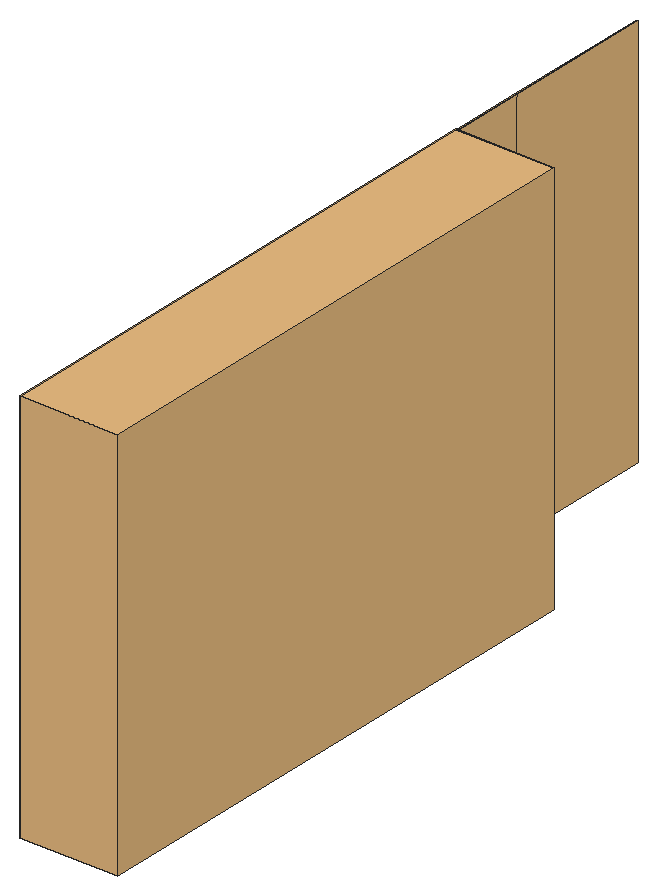
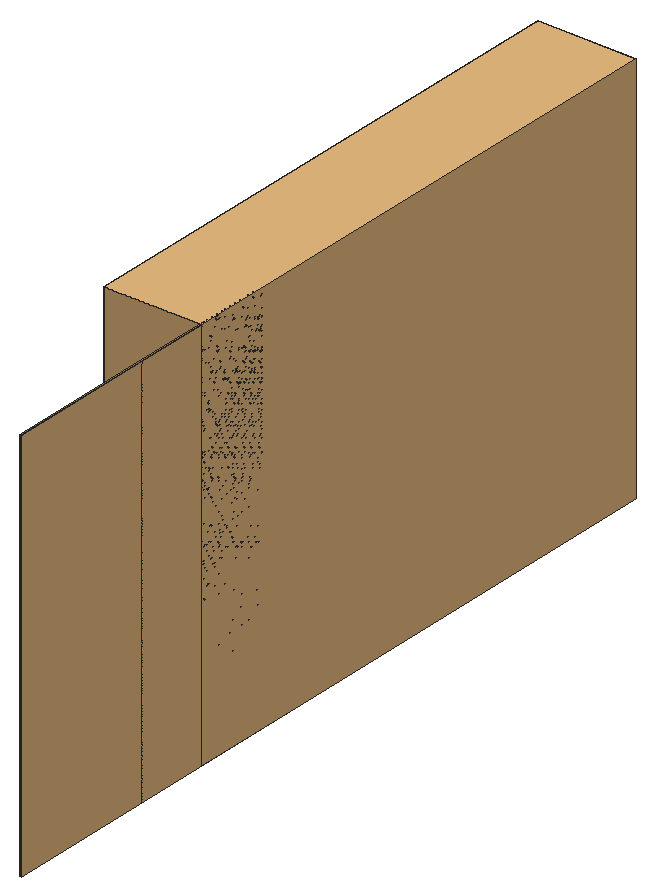
# SketchUp Ruby script. Lengths in inches.
U = 1.inch
M = Sketchup.active_model
def pt(a) = Geom::Point3d.new(a.map { |v| v * U })
def face(e, loops, mat)
  f = e.add_face(loops[0].map { |a| pt(a) })
  loops[1..].each { |l| e.add_face(l.map { |a| pt(a) }).erase! }
  f.material = f.back_material = mat if mat
  f
end
# faces: each face lists its corners as indices into pts; further lists are holes
def faces(e, pts, list, mat = nil) = list.each { |f| face(e, (f[0].is_a?(Array) ? f : [f]).map { |l| l.map { |i| pts[i] } }, mat) }
# xy, xz, yz: faces in a plane at the given z, y or x. An outline is a flat list of corners, or four numbers for a rectangle; further outlines are holes
def ring(l) = l.size == 4 ? [[l[0], l[1]], [l[2], l[1]], [l[2], l[3]], [l[0], l[3]]] : l.each_slice(2).to_a
def flat(e, list, mat, &to3) = list.each { |f| face(e, (f[0].is_a?(Array) ? f : [f]).map { |l| ring(l).map { |u, v| to3.(u, v) } }, mat) }
def xy(e, z, list, mat = nil) = flat(e, list, mat) { |x, y| [x, y, z] }
def xz(e, y, list, mat = nil) = flat(e, list, mat) { |x, z| [x, y, z] }
def yz(e, x, list, mat = nil) = flat(e, list, mat) { |y, z| [x, y, z] }
def lines(e, pts, list) = list.each { |a, b| e.add_line(pt(pts[a]), pt(pts[b])) }
# prism: a flat outline (further loops are holes) pulled along v
def prism(e, loops, v, mat = nil)
  f = face(e, loops, mat); d = Geom::Vector3d.new(v.map { |x| x * U })
  f.pushpull(f.normal.samedirection?(d) ? d.length : -d.length)
end
def box(e, o, s, mat = nil) = prism(e, [[o, [o[0] + s[0], o[1], o[2]], [o[0] + s[0], o[1] + s[1], o[2]], [o[0], o[1] + s[1], o[2]]]], [0, 0, s[2]], mat)
def at(x, y, z, deg = 0) = Geom::Transformation.translation(pt([x, y, z])) * Geom::Transformation.rotation(ORIGIN, Z_AXIS, deg.degrees)
def axes(o, x, y, z) = Geom::Transformation.new([*x, 0, *y, 0, *z, 0, *pt(o).to_a, 1])
def part(name) = M.definitions.add(name)
# library, detail: a bought-in or finely detailed component or shape, given as its bounding box
def library(name, o, s) = part(name).tap { |d| box(d.entities, o, s) }
def detail(e, o, s) = box(e.add_group.entities, o, s)
def put(e, d, t, mat = nil) = e.add_instance(d, t).tap { |i| i.material = mat if mat }
def group(e, t, mat = nil) = e.add_group.tap { |g| g.transformation = t; g.material = mat if mat }.entities
root = M.entities
M.materials.add("[Wood Veneer 01]").color = [120, 70, 37]
M.materials.add("green").color = [174, 139, 102]
M.materials.add("vio").color = [206, 114, 100]
c1 = library("3DGeom~53_Defintion",[-197.77,-500,-314.82],[395.54,1000,629.64])
c2 = part("3DGeom~54_Defintion")
p = [[-142.75,-484.5,-308.47],[-174.69,-472.9,-312.45],[-157.62,-477.6,-314.82],[-174.69,-472.9,-312.45],[-142.75,-484.5,-308.47],[-197.77,-474.24,-286.23],
  [-174.69,-472.9,-312.45],[-197.77,-474.24,-286.23],[-189.38,-471.68,-301.98],[-188.9,-487.18,-256.03],[-142.75,-484.5,-308.47],[-156.97,-498.77,-252.06],
  [-156.97,-498.77,-252.06],[-142.75,-484.5,-308.47],[-133.89,-497.43,-278.27],[-142.75,-484.5,-308.47],[-134.07,-491.76,-295.09],[-133.89,-497.43,-278.27],
  [-197.77,-474.24,-286.23],[-142.75,-484.5,-308.47],[-188.9,-487.18,-256.03],[-197.77,-474.24,-286.23],[-188.9,-487.18,-256.03],[-197.59,-479.92,-269.41],
  [-156.97,-498.77,-252.06],[-133.89,-497.43,-278.27],[-142.27,-500,-262.52],[-188.9,-487.18,-256.03],[-156.97,-498.77,-252.06],[-174.04,-494.08,-249.68],
  [187.69,494.74,272.45],[154.39,500,263.8],[138.33,494.89,269.58],[187.69,494.74,272.45],[172.46,499.94,264.85],[154.39,500,263.8],
  [187.69,494.74,272.45],[138.33,494.89,269.58],[128.58,485.99,280.65],[187.69,494.74,272.45],[136.08,466.72,306.16],[151.32,461.51,313.77],
  [187.69,494.74,272.45],[169.38,461.46,314.82],[187.69,494.74,272.45],[185.44,466.57,309.04],[187.69,494.74,272.45],[185.44,466.57,309.04],
  [195.19,475.47,297.97],[187.69,494.74,272.45],[127.76,475.68,294.04],[187.69,494.74,272.45],[195.19,475.47,297.97],[196.01,485.78,284.58],
  [187.69,494.74,272.45],[128.58,485.99,280.65],[127.76,475.68,294.04]]
faces(c2.entities,p,[[0,1,2],[3,4,5],[6,7,8],[9,10,11],[12,13,14],[15,16,17],[18,19,20],[21,22,23],
  [24,25,26],[27,28,29],[30,31,32],[33,34,35],[36,37,38],[39,40,41],[42,41,43],[44,43,45],
  [46,47,48],[49,50,40],[51,52,53],[54,55,56]],"green")
c3 = part("3DGeom~200_Defintion")
p = [[-43.89,-289.91,-363.15],[-189.17,-120.3,-441.1],[-12.44,-14.18,-500],[160.18,-167.375,-431.16],[127.12,130.77,-458.85],[-181.73,142.8125,-434.86],
  [-101.15,226.5,-411.11],[321.33,0,-383.65],[321.33,0,-383.65],[192.11,275.72,-328.68],[-63.63,310.1875,-335.95],[-63.63,310.1875,-335.95],
  [192.11,275.72,-328.68],[-236.2,-334.76,-197.83],[-355.71,-159.14,-297.93],[-236.2,-334.76,-197.83],[-355.71,-159.14,-297.93],[-283.76,81.55,-400.86],
  [-302.32,261.54,-253.21],[-302.32,261.54,-253.21],[113.15,-381.84,-187.89],[113.15,-381.84,-187.89],[289.875,-275.72,-246.79],[289.875,-275.72,-246.79],
  [321.33,0,-383.65],[-63.63,310.1875,-335.95],[-302.32,261.54,-253.21],[-355.71,-159.14,-297.93],[-379.91,59.12,-318.2],[-283.76,81.55,-400.86],
  [-379.91,59.12,-318.2],[-302.32,261.54,-253.21],[289.875,-275.72,-246.79],[321.33,0,-383.65],[429.43,-130.77,-205.64],[429.43,-130.77,-205.64],
  [321.33,0,-383.65],[396.375,167.38,-233.33],[321.33,0,-383.65],[192.11,275.72,-328.68],[396.375,167.38,-233.33],[-53.39,-420.67,-44.72],
  [-236.2,-334.76,-197.83],[-43.89,-289.91,-363.15],[-43.89,-289.91,-363.15],[113.15,-381.84,-187.89],[-79.21,371.45,-229.53],[-63.63,310.1875,-335.95],
  [-302.32,261.54,-253.21],[192.11,275.72,-328.68],[192.11,275.72,-328.68],[165.125,381.84,-144.36],[192.11,275.72,-328.68],[165.125,381.84,-144.36],
  [-467.44,-120.3,-108.85],[-355.71,-159.14,-297.93],[-444.42,81.55,-209.03],[-365.21,-289.91,20.5],[-236.2,-334.76,-197.83],[-365.21,-289.91,20.5],
  [-460,142.8125,-102.62],[-422.48,226.5,-27.46],[-341.9,310.1875,-3.7],[-341.9,310.1875,-3.7],[-239.87,371.45,-37.71],[-302.32,261.54,-253.21],
  [-143.72,393.875,-120.37],[-302.32,261.54,-253.21],[-302.32,261.54,-253.21],[239.87,-371.45,37.71],[289.875,-275.72,-246.79],[289.875,-275.72,-246.79],
  [341.9,-310.19,3.7],[341.9,-310.19,3.7],[289.875,-275.72,-246.79],[494.43,14.18,-75.47],[365.21,289.91,-20.5],[165.125,381.84,-144.36],
  [-494.43,-14.18,75.47],[422.48,-226.5,27.46],[-165.125,-381.83,144.36],[-365.21,-289.91,20.5],[143.72,-393.875,120.37],[365.21,289.91,-20.5],
  [53.39,420.68,44.72],[-396.375,-167.375,233.33],[-365.21,-289.91,20.5],[-429.43,130.77,205.64],[460,-142.8125,102.62],[467.44,120.3,108.85],
  [79.21,-371.45,229.53],[-113.15,381.83,187.89],[-341.9,310.1875,-3.7],[-113.15,381.83,187.89],[-289.875,275.72,246.79],[-289.875,275.72,246.79],
  [236.2,334.75,197.83],[365.21,289.91,-20.5],[236.2,334.75,197.83],[-113.15,381.83,187.89],[-341.9,310.1875,-3.7],[-289.875,275.72,246.79],
  [341.9,-310.19,3.7],[302.32,-261.54,253.21],[302.32,-261.54,253.21],[-192.11,-275.72,328.68],[-365.21,-289.91,20.5],[-165.125,-381.83,144.36],
  [-192.11,-275.72,328.68],[-365.21,-289.91,20.5],[302.32,-261.54,253.21],[236.2,334.75,197.83],[-113.15,381.83,187.89],[-321.32,0,383.65],
  [-321.32,0,383.65],[444.42,-81.55,209.03],[302.32,-261.54,253.21],[355.71,159.14,297.93],[236.2,334.75,197.83],[355.71,159.14,297.93],
  [63.63,-310.1875,335.95],[-192.11,-275.72,328.68],[43.89,289.91,363.15],[-113.15,381.83,187.89],[-289.875,275.72,246.79],[236.2,334.75,197.83],
  [-113.15,381.83,187.89],[43.89,289.91,363.15],[355.71,159.14,297.93],[236.2,334.75,197.83],[-160.18,167.375,431.16],[-429.43,130.77,205.64],
  [-321.32,0,383.65],[-429.43,130.77,205.64],[379.91,-59.12,318.2],[302.32,-261.54,253.21],[355.71,159.14,297.93],[-127.12,-130.77,458.85],
  [-396.375,-167.375,233.33],[-192.11,-275.72,328.68],[-396.375,-167.375,233.33],[101.15,-226.5,411.11],[63.63,-310.1875,335.95],[302.32,-261.54,253.21],
  [181.73,-142.8125,434.86],[302.32,-261.54,253.21],[283.76,-81.55,400.86],[302.32,-261.54,253.21],[283.76,-81.55,400.86],[302.32,-261.54,253.21],
  [379.91,-59.12,318.2],[189.17,120.3,441.1],[379.91,-59.12,318.2],[-192.11,-275.72,328.68],[63.63,-310.1875,335.95],[-192.11,-275.72,328.68],
  [12.44,14.18,500]]
faces(c3.entities,p,[[0,1,2],[0,2,3],[3,2,4],[1,5,2],[2,5,6],[2,6,4],[3,4,7],[8,4,9],
  [4,6,10],[4,11,12],[13,14,1],[15,1,0],[16,17,1],[1,17,5],[5,17,18],[6,5,19],
  [20,0,3],[21,3,22],[23,3,24],[25,6,26],[27,28,17],[29,30,31],[32,33,34],[35,36,37],
  [38,39,40],[41,42,43],[41,44,45],[46,47,48],[49,47,46],[37,50,51],[52,46,53],[54,30,55],
  [54,56,30],[30,56,31],[57,55,58],[59,54,55],[56,60,31],[60,61,31],[61,62,31],[63,64,65],
  [64,66,67],[66,46,68],[69,45,70],[69,71,72],[73,74,35],[35,37,75],[75,37,76],[37,77,76],
  [53,46,66],[78,56,54],[78,60,56],[73,35,79],[79,35,75],[80,42,41],[80,81,42],[82,41,45],
  [82,45,69],[83,53,84],[53,66,84],[84,66,64],[85,54,86],[85,78,54],[87,60,78],[87,61,60],
  [79,75,88],[88,75,89],[75,76,89],[90,80,41],[90,41,82],[91,64,92],[84,64,93],[94,61,87],
  [95,62,61],[89,76,96],[97,84,98],[99,100,101],[69,102,103],[73,79,104],[105,106,107],[108,85,109],
  [79,88,110],[82,69,103],[111,84,112],[113,78,85],[114,87,78],[88,115,116],[88,89,115],[115,89,117],
  [89,118,119],[90,82,103],[120,121,80],[120,80,90],[122,123,124],[125,126,127],[128,129,122],[130,131,132],
  [130,124,133],[115,134,135],[115,136,134],[120,90,103],[137,138,139],[137,132,140],[122,124,130],[141,142,143],
  [144,141,145],[146,144,147],[134,148,149],[150,128,151],[128,122,151],[152,151,146],[141,153,154],[141,137,155],
  [151,122,130],[156,132,137],[156,130,132],[146,156,144],[146,151,156],[144,137,141],[151,130,156],[144,156,137]],"vio")
c4 = part("3DGeom~207_Defintion")
p = [[-123.67,-51.48,-497.34],[-293.26,-262.53,-290.98],[-357.11,-52.125,-367.46],[-91.11,-261.97,-403.46],[-293.26,-262.53,-290.98],[142.89,-37.04,-493.96],
  [-123.1,172.81,-457.96],[-357.11,-52.125,-367.46],[107.75,185.3125,-455.03],[139.75,-249.46,-400.53],[371.18,-12.67,-358.22],[305.45,206.42,-337.48],
  [305.45,206.42,-337.48],[371.18,-12.67,-358.22],[-357.11,-52.125,-367.46],[-325.26,172.25,-345.47],[-89.55,350.79,-295.86],[-325.26,172.25,-345.47],
  [43.74,358.01,-294.17],[43.74,358.01,-294.17],[-89.55,350.79,-295.86],[157.88,370.19,-226.31],[43.74,358.01,-294.17],[157.88,370.19,-226.31],
  [305.45,206.42,-337.48],[-91.11,-261.97,-403.46],[-150.84,-402.59,-136.53],[-293.26,-262.53,-290.98],[-91.11,-261.97,-403.46],[-34.13,-402.27,-201.48],
  [139.75,-249.46,-400.53],[-91.11,-261.97,-403.46],[139.75,-249.46,-400.53],[99.16,-395.05,-199.79],[337.45,-228.36,-282.98],[139.75,-249.46,-400.53],
  [371.18,-12.67,-358.22],[337.45,-228.36,-282.98],[-357.11,-52.125,-367.46],[-293.26,-262.53,-290.98],[-412.55,-251,-93.23],[-494.85,-38.81,-139.11],
  [-325.26,172.25,-345.47],[500,15.09,-126.5],[337.45,-228.36,-282.98],[371.18,-12.67,-358.22],[417.02,230.46,-136.8],[305.45,206.42,-337.48],
  [417.02,230.46,-136.8],[-444.55,183.78,-147.72],[-206.26,350.47,-230.92],[-89.55,350.79,-295.86],[-325.26,172.25,-345.47],[-206.26,350.47,-230.92],
  [222.29,384.07,-110.45],[305.45,206.42,-337.48],[157.88,370.19,-226.31],[417.02,230.46,-136.8],[-89.55,350.79,-295.86],[-206.26,350.47,-230.92],
  [-32,434.78,-54.5],[43.74,358.01,-294.17],[-293.26,-262.53,-290.98],[-219.72,-395.93,-22.36],[-293.26,-262.53,-290.98],[-219.72,-395.93,-22.36],
  [-412.55,-251,-93.23],[337.45,-228.36,-282.98],[213.3,-382.87,-131.92],[449.01,-204.32,-82.31],[213.3,-382.87,-131.92],[-206.26,350.47,-230.92],
  [-275.13,357.125,-116.75],[-275.13,357.125,-116.75],[32,-434.78,54.5],[213.3,-382.87,-131.92],[-500,-15.09,126.5],[-449.01,204.32,82.31],
  [-275.13,357.125,-116.75],[-417.02,-230.46,136.8],[412.55,251,93.23],[417.02,230.46,-136.8],[219.72,395.93,22.36],[417.02,230.46,-136.8],
  [219.72,395.93,22.36],[417.02,230.46,-136.8],[222.29,384.07,-110.45],[-219.72,-395.93,-22.36],[213.3,-382.87,-131.92],[277.71,-368.99,-16.06],
  [277.71,-368.99,-16.06],[494.85,38.81,139.12],[-275.13,357.125,-116.75],[-277.71,368.99,16.06],[-277.71,368.99,16.06],[219.72,395.93,22.36],
  [-219.72,-395.93,-22.36],[-222.29,-384.07,110.45],[-222.29,-384.07,110.45],[444.55,-183.78,147.72],[-213.3,382.87,131.92],[-99.16,395.05,199.79],
  [34.13,402.27,201.48],[150.84,402.59,136.53],[-222.29,-384.07,110.45],[-219.72,-395.93,-22.36],[277.71,-368.99,-16.06],[275.13,-357.125,116.75],
  [275.13,-357.125,116.75],[-277.71,368.99,16.06],[-337.45,228.36,282.98],[-277.71,368.99,16.06],[-337.45,228.36,282.98],[-213.3,382.87,131.92],
  [412.55,251,93.23],[-157.88,-370.19,226.31],[-43.74,-358.01,294.17],[-157.88,-370.19,226.31],[89.55,-350.79,295.86],[-43.74,-358.01,294.17],
  [275.13,-357.125,116.75],[206.26,-350.47,230.92],[206.26,-350.47,230.92],[89.55,-350.79,295.86],[-371.18,12.67,358.22],[-371.18,12.67,358.22],
  [-337.45,228.36,282.98],[293.26,262.53,290.98],[293.26,262.53,290.98],[412.55,251,93.23],[-417.02,-230.46,136.8],[-157.88,-370.19,226.31],
  [325.26,-172.25,345.47],[206.26,-350.47,230.92],[-305.45,-206.42,337.48],[-305.45,-206.42,337.48],[-371.18,12.67,358.22],[-337.45,228.36,282.98],
  [-139.75,249.46,400.53],[-417.02,-230.46,136.8],[-157.88,-370.19,226.31],[-305.45,-206.42,337.48],[357.1,52.125,367.46],[293.26,262.53,290.98],
  [91.11,261.97,403.46],[-305.45,-206.42,337.48],[-157.88,-370.19,226.31],[-43.74,-358.01,294.17],[123.1,-172.81,457.96],[89.55,-350.79,295.86],
  [206.26,-350.47,230.92],[206.26,-350.47,230.92],[325.26,-172.25,345.47],[-337.45,228.36,282.98],[-371.18,12.67,358.22],[-142.9,37.04,493.96],
  [-337.45,228.36,282.98],[-139.75,249.46,400.53],[91.11,261.97,403.46],[357.1,52.125,367.46],[293.26,262.53,290.98],[-107.75,-185.3125,455.03],
  [123.67,51.48,497.34],[325.26,-172.25,345.47],[325.26,-172.25,345.47],[357.1,52.125,367.46],[91.11,261.97,403.46],[357.1,52.125,367.46],
  [-139.75,249.46,400.53],[-139.75,249.46,400.53],[91.11,261.97,403.46]]
faces(c4.entities,p,[[0,1,2],[0,3,4],[5,3,0],[6,0,7],[8,5,0],[8,0,6],[5,9,3],[10,9,5],
  [11,5,8],[12,13,5],[6,14,15],[16,6,17],[18,8,6],[19,6,20],[21,8,22],[23,24,8],
  [25,26,27],[28,29,26],[30,29,31],[32,33,29],[34,33,35],[36,37,9],[38,39,40],[38,40,41],
  [42,38,41],[43,44,45],[46,45,47],[48,43,45],[42,41,49],[50,42,49],[51,52,53],[54,55,56],
  [54,57,55],[58,59,60],[61,58,60],[56,61,60],[62,26,63],[64,65,66],[67,68,33],[69,70,44],
  [43,69,44],[71,49,72],[59,73,60],[54,56,60],[26,29,74],[29,33,74],[33,75,74],[49,41,76],
  [49,76,77],[78,49,77],[41,40,79],[41,79,76],[80,43,81],[82,80,83],[84,85,86],[87,26,74],
  [88,89,74],[69,90,70],[91,69,43],[80,91,43],[92,77,93],[73,94,60],[95,54,60],[40,96,97],
  [40,98,79],[99,90,69],[91,99,69],[94,100,60],[100,101,60],[101,102,60],[103,95,60],[102,103,60],
  [104,105,74],[106,107,74],[99,108,90],[109,77,110],[111,112,113],[103,114,95],[115,104,74],[116,117,74],
  [118,119,74],[120,121,74],[122,123,74],[77,76,124],[77,125,126],[127,91,80],[103,128,129],[130,104,131],
  [132,133,108],[132,108,99],[76,79,134],[76,135,136],[100,137,138],[100,138,101],[102,128,103],[139,140,141],
  [142,99,91],[143,142,91],[142,132,99],[101,138,144],[101,144,102],[102,144,128],[145,146,147],[148,149,150],
  [148,151,152],[153,154,155],[156,155,157],[158,159,160],[145,147,161],[161,147,149],[161,149,148],[154,145,161],
  [162,148,163],[162,164,165],[154,161,155],[166,162,167],[168,155,162],[169,162,170],[155,161,148],[155,148,162]],"vio")
c5 = part("3DGeom~29_Defintion")
p = [[-0.99,-278.38,-126.59],[-1.52,-278.38,-126.5],[-1.54,-300.55,-125.92],[-1.03,-300.56,-126.01],[-0.92,-237.29,-119.72],[-1.49,-257.76,-123.95],
  [-0.93,-257.75,-124.05],[-1.51,-237.3,-119.62],[-1.01,-325.68,-120.9],[-1.49,-325.66,-120.82],[-1.39,-353.61,-111.43],[-0.95,-353.63,-111.5],
  [-1.3,-191.54,-111.3],[-1.63,-215.67,-114.9],[-1.03,-215.65,-115],[-1.93,-191.55,-111.2],[-3.02,-132.81,-105.31],[-2.625,-163.72,-108.34],
  [-1.96,-163.7,-108.45],[-3.72,-132.84,-105.1875],[-5.18,-69.94,-97.84],[-4.92,-100.91,-101.67],[-4.19,-100.88,-101.79],[-5.9375,-69.97,-97.71],
  [-0.875,-383.21,-98.93],[-1.28,-383.1875,-98.87],[-1.16,-414.39,-83.14],[-0.79,-414.41,-83.19],[-5.45,-19.25,-88.36],[-6.48,-42.06,-93.25],
  [-5.69,-42.04,-93.38],[-6.27,-19.26,-88.22],[-1.87,9.64,-75.67],[-4.96,-2.54,-82.33],[-4.125,-2.57,-82.49],[-2.71,9.7,-75.49],
  [3.6,27.06,-60.84],[0,19.07,-68.14],[0.85,18.99,-68.34],[2.74,27.13,-60.65],[-0.7,-447.22,-64.28],[-1.03,-447.2,-64.23],
  [-0.89,-481.62,-42.16],[-0.6,-481.64,-42.21],[7.12,45.46,-47.33],[5,35.43,-53.44],[5.89,35.39,-53.61],[6.21,45.44,-47.2],
  [5.77,67.15,-39.5],[6.03,56.38,-42.66],[6.95,56.45,-42.77],[4.84,67.03,-39.4],[2.28,88.125,-34.02],[3.13,77.53,-36.72],
  [4.07,77.66,-36.82],[1.33,87.99,-33.92],[0.14,109.59,-25.46],[-0.13,98.6,-30.34],[0.84,98.7,-30.46],[-0.84,109.53,-25.32],
  [1.14,134.61,-9.66],[-0.65,121.53,-18.23],[0.34,121.57,-18.38],[0.13,134.59,-9.49],[3.45,160.94,9.61],[1.25,147.95,0.1],
  [2.27,147.97,-0.07],[2.41,160.92,9.78],[4.85,182.93,26.1875],[3.35,172.78,18.77],[4.4,172.82,18.61],[3.78,182.86,26.33],
  [4,196.81,36.55],[3.57,190.65,32.07],[4.65,190.76,31.96],[2.91,196.65,36.625],[2.24,206.05,44],[2.03,201.51,40.46],
  [3.12,201.7,40.41],[1.14,205.87,44.0625],[1.32,215.82,52.37],[0.46,210.4,47.92],[1.57,210.54,47.82],[0.2,215.73,52.51],
  [2.32,227.77,63.67],[0.49,221.62,57.88],[1.61,221.67,57.7],[1.19,227.73,63.87],[4.19,240.64,76.25],[2.11,234.07,70.16],
  [3.25,234.09,69.95],[3.05,240.61,76.46],[5.3,254.43,87.65],[3.79,247.37,82.45],[4.95,247.41,82.25],[4.13,254.36,87.82],
  [4.65,267.57,96.37],[3.97,260.98,92.36],[5.15,261.09,92.21],[3.47,267.43,96.5],[3.1875,281.38,103.64],[2.75,274.07,100.29],
  [3.95,274.22,100.16],[1.98,281.25,103.78],[2.11,298.65,109.88],[1.3125,289.3125,107.01],[2.53,289.41,106.86],[0.89,298.59,110.05],
  [1.95,318.85,115.22],[0.72,308.52,112.86],[1.96,308.5625,112.68],[0.7,318.83,115.4],[2.17,342.62,119.6],[0.77,330.02,117.71],
  [2.04,330.04,117.52],[0.89,342.6,119.79],[2.37,374.03,123.25],[1,357.1,121.69],[2.29,357.11,121.5],[1.0625,374.02,123.44],
  [2.46,414.46,126.33],[1.08,393.28,125.07],[2.42,393.29,124.875],[1.1,414.46,126.53],[2.55,462.57,128.68],[1.12,437.55,127.8],
  [2.51,437.56,127.59],[1.13,462.5625,128.89],[2.62,518.36,130.3125],[1.14,489.5,129.8],[2.58,489.5,129.59],[1.15,518.36,130.53]]
faces(c5.entities,p,[[0,1,2],[0,2,3],[4,5,6],[4,7,5],[8,9,10],[8,10,11],[12,13,14],[12,15,13],
  [16,17,18],[16,19,17],[20,21,22],[20,23,21],[24,25,26],[24,26,27],[28,29,30],[28,31,29],
  [32,33,34],[32,35,33],[36,37,38],[36,39,37],[40,41,42],[40,42,43],[44,45,46],[44,47,45],
  [48,49,50],[48,51,49],[52,53,54],[52,55,53],[56,57,58],[56,59,57],[60,61,62],[60,63,61],
  [64,65,66],[64,67,65],[68,69,70],[68,71,69],[72,73,74],[72,75,73],[76,77,78],[76,79,77],
  [80,81,82],[80,83,81],[84,85,86],[84,87,85],[88,89,90],[88,91,89],[92,93,94],[92,95,93],
  [96,97,98],[96,99,97],[100,101,102],[100,103,101],[104,105,106],[104,107,105],[108,109,110],[108,111,109],
  [112,113,114],[112,115,113],[116,117,118],[116,119,117],[120,121,122],[120,123,121],[124,125,126],[124,127,125],
  [128,129,130],[128,131,129]],"green")
c6 = part("3DGeom~30_Defintion")
p = [[-0.92,-255.91,-123.16],[-1.51,-276.4,-125.6],[-0.98,-276.4,-125.69],[-1.48,-255.93,-123.07],[-1.03,-298.42,-125.11],[-1.48,-323.34,-119.96],
  [-1.01,-323.36,-120.04],[-1.53,-298.41,-125.02],[-1.02,-214.12,-114.1875],[-1.5,-235.61,-118.77],[-0.92,-235.6,-118.87],[-1.62,-214.14,-114.08],
  [-0.94,-351.11,-110.71],[-1.38,-351.09,-110.63],[-1.27,-380.46,-98.16],[-0.87,-380.48,-98.23],[-1.95,-162.54,-107.68],[-1.92,-190.19,-110.4],
  [-1.29,-190.18,-110.51],[-2.61,-162.56,-107.57],[-4.16,-100.16,-101.07],[-3.69,-131.89,-104.44],[-3,-131.86,-104.56],[-4.88,-100.1875,-100.95],
  [-5.65,-41.74,-92.72],[-5.89,-69.47,-97.02],[-5.14,-69.44,-97.15],[-6.4375,-41.76,-92.58],[-4.1,-2.55,-81.9],[-6.23,-19.12,-87.59],
  [-5.41,-19.11,-87.73],[-4.92,-2.52,-81.75],[-0.79,-411.46,-82.6],[-1.15,-411.43,-82.54],[-1.02,-444.01,-63.78],[-0.7,-444.04,-63.83],
  [0.85,18.85,-67.85],[-2.6875,9.63,-74.96],[-1.85,9.58,-75.14],[0,18.93,-67.66],[5.85,35.14,-53.23],[2.72,26.94,-60.21],
  [3.58,26.86,-60.41],[4.97,35.17,-53.0625],[6.9,56.05,-42.47],[6.17,45.12,-46.86],[7.07,45.14,-46.99],[5.98,55.98,-42.36],
  [-0.6,-478.21,-41.9],[-0.88,-478.19,-41.86],[-0.73,-513.97,-16.8],[-0.49,-513.98,-16.83],[4.04,77.11,-36.55],[4.81,66.56,-39.12],
  [5.73,66.67,-39.22],[3.11,76.97,-36.46],[0.83,98,-30.24],[1.32,87.37,-33.68],[2.26,87.5,-33.78],[-0.13,97.9,-30.13],
  [0.34,120.7,-18.25],[-0.83,108.75,-25.14],[0.14,108.81,-25.28],[-0.65,120.67,-18.1],[2.26,146.92,-0.07],[0.13,133.625,-9.43],
  [1.14,133.65,-9.59],[1.24,146.9,0.1],[4.375,171.59,18.48],[2.39,159.77,9.71],[3.43,159.79,9.54],[3.32,171.55,18.64],
  [4.62,189.41,31.74],[3.75,181.5625,26.14],[4.82,181.63,26],[3.54,189.29,31.85],[3.1,200.26,40.12],[2.89,195.25,36.37],
  [3.97,195.41,36.29],[2.02,200.07,40.17],[1.56,209.04,47.48],[0.46,208.9,47.58],[1.14,204.4,43.75],[2.22,204.59,43.6875],
  [1.6,220.09,57.29],[0.2,214.2,52.14],[1.31,214.28,51.99],[0.49,220.04,57.47],[3.23,232.43,69.45],[1.18,226.11,63.41],
  [2.31,226.15,63.21],[2.1,232.4,69.66],[4.92,245.65,81.67],[3.02,238.9,75.91],[4.17,238.93,75.71],[3.77,245.61,81.86],
  [5.12,259.24,91.55],[4.1,252.55,87.19],[5.27,252.62,87.02],[3.95,259.12,91.7],[3.92,272.26,99.45],[3.44,265.52,95.8125],
  [4.62,265.66,95.68],[2.73,272.12,99.58],[2.51,287.35,106.1],[1.97,279.25,103.04],[3.16,279.38,102.9],[1.3,287.25,106.25],
  [1.95,306.36,111.88],[0.88,296.47,109.26],[2.1,296.52,109.1],[0.72,306.32,112.05],[2.02,327.68,116.68],[0.69,316.56,114.58],
  [1.9375,316.58,114.4],[0.76,327.67,116.87],[2.28,354.5625,120.64],[0.88,340.16,118.94],[2.15,340.18,118.75],[0.99,354.55,120.83],
  [2.4,390.49,123.99],[1.05,371.36,122.5625],[2.35,371.37,122.37],[1.07,390.48,124.18],[2.49,434.4375,126.68],[1.09,411.5,125.625],
  [2.44,411.51,125.43],[1.11,434.43,126.89],[2.57,486.02,128.66],[1.125,459.27,127.97],[2.53,459.27,127.76],[1.14,486.01,128.875]]
faces(c6.entities,p,[[0,1,2],[0,3,1],[4,5,6],[4,7,5],[8,9,10],[8,11,9],[12,13,14],[12,14,15],
  [16,17,18],[16,19,17],[20,21,22],[20,23,21],[24,25,26],[24,27,25],[28,29,30],[28,31,29],
  [32,33,34],[32,34,35],[36,37,38],[36,39,37],[40,41,42],[40,43,41],[44,45,46],[44,47,45],
  [48,49,50],[48,50,51],[52,53,54],[52,55,53],[56,57,58],[56,59,57],[60,61,62],[60,63,61],
  [64,65,66],[64,67,65],[68,69,70],[68,71,69],[72,73,74],[72,75,73],[76,77,78],[76,79,77],
  [80,81,82],[80,82,83],[84,85,86],[84,87,85],[88,89,90],[88,91,89],[92,93,94],[92,95,93],
  [96,97,98],[96,99,97],[100,101,102],[100,103,101],[104,105,106],[104,107,105],[108,109,110],[108,111,109],
  [112,113,114],[112,115,113],[116,117,118],[116,119,117],[120,121,122],[120,123,121],[124,125,126],[124,127,125],
  [128,129,130],[128,131,129]],"green")
c7 = library("3DGeom~31_Defintion",[-9.58,-482.04,-130.39],[19.16,1000,260.06])
c8 = library("3DGeom~32_Defintion",[-7.28,-481.66,-126.81],[15.21,1000,257.33])
c9 = library("3DGeom~33_Defintion",[-9.51,-514.28,-129.47],[19.02,1000,257.51])
c10 = library("3DGeom~34_Defintion",[-7.23,-514,-125.91],[15.11,1000,254.78])
c11 = library("3DGeom~35_Defintion",[-9.58,-482.04,-130.39],[19.16,1000,260.6])
c12 = library("3DGeom~36_Defintion",[-9.51,-514.28,-129.47],[19.02,1000,258.04])
c13 = part("3DGeom~37_Defintion")
p = [[-0.78,-500,-17.86],[-0.32,-499.95,-17.77],[-1.37,-499.29,-16.52],[-1.24,-499.9375,-17.74],[-0.78,-500,-17.86],[-1.37,-499.29,-16.52],
  [-1.24,-499.9375,-17.74],[-1.02,-499.98,-17.83],[-0.78,-500,-17.86],[-0.78,-500,-17.86],[-0.54,-499.99,-17.84],[-0.32,-499.95,-17.77],
  [-0.32,-499.95,-17.77],[0.02,-499.81,-17.51],[-1.37,-499.29,-16.52],[-0.32,-499.95,-17.77],[-0.13,-499.89,-17.66],[0.02,-499.81,-17.51],
  [-1.52,-499.375,-16.67],[-1.42,-499.87,-17.61],[-1.24,-499.9375,-17.74],[-1.52,-499.375,-16.67],[-1.24,-499.9375,-17.74],[-1.37,-499.29,-16.52],
  [-1.64,-499.6875,-17.26],[-1.55,-499.79,-17.45],[-1.42,-499.87,-17.61],[-1.64,-499.6875,-17.26],[-1.42,-499.87,-17.61],[-1.52,-499.375,-16.67],
  [0.02,-499.81,-17.51],[0.16,-499.6,-17.12],[-1.37,-499.29,-16.52],[0.02,-499.81,-17.51],[0.12,-499.71,-17.32],[0.16,-499.6,-17.12],
  [-1.52,-499.375,-16.67],[-1.66,-499.58,-17.06],[-1.64,-499.6875,-17.26],[-1.52,-499.375,-16.67],[-1.62,-499.47,-16.85],[-1.66,-499.58,-17.06],
  [0.16,-499.6,-17.12],[0.06,-499.4,-16.72],[-1.37,-499.29,-16.52],[0.16,-499.6,-17.12],[0.14,-499.5,-16.91],[0.06,-499.4,-16.72],
  [0.06,-499.4,-16.72],[-0.26,-499.25,-16.4375],[-1.37,-499.29,-16.52],[0.06,-499.4,-16.72],[-0.08,-499.3125,-16.5625],[-0.26,-499.25,-16.4375],
  [-0.71,-499.18,-16.3125],[-1.18,-499.23,-16.4],[-1.37,-499.29,-16.52],[-0.26,-499.25,-16.4375],[-0.71,-499.18,-16.3125],[-1.37,-499.29,-16.52],
  [-0.71,-499.18,-16.3125],[-0.96,-499.19,-16.33],[-1.18,-499.23,-16.4],[-0.26,-499.25,-16.4375],[-0.47,-499.2,-16.35],[-0.71,-499.18,-16.3125],
  [0.97,500,115.21],[-2.68,499.88,124.36],[3.67,499.99,115.9],[-1.71,499.99,115.97],[-2.68,499.88,124.36],[0.97,500,115.21],
  [-1.71,499.99,115.97],[0.97,500,115.21],[-0.44,500,115.42],[0.97,500,115.21],[3.67,499.99,115.9],[2.39,500,115.38],
  [3.67,499.99,115.9],[-2.68,499.88,124.36],[5.61,499.97,117.79],[3.67,499.99,115.9],[5.61,499.97,117.79],[4.76,499.98,116.72],
  [-3.53,499.9,123.29],[-2.68,499.88,124.36],[-1.71,499.99,115.97],[-3.53,499.9,123.29],[-1.71,499.99,115.97],[-2.78,499.98,116.82],
  [-4.12,499.95,119.1875],[-3.53,499.9,123.29],[-2.78,499.98,116.82],[-4.12,499.95,119.1875],[-2.78,499.98,116.82],[-3.6,499.97,117.91],
  [5.61,499.97,117.79],[-2.68,499.88,124.36],[6.375,499.93,120.47],[5.61,499.97,117.79],[6.375,499.93,120.47],[6.17,499.95,119.06],
  [-4.29,499.93,120.61],[-3.53,499.9,123.29],[-4.12,499.95,119.1875],[6.375,499.93,120.47],[-2.68,499.88,124.36],[5.68,499.9,123.17],
  [6.375,499.93,120.47],[5.68,499.9,123.17],[6.2,499.91,121.89],[-4.29,499.93,120.61],[-4.08,499.91,122.02],[-3.53,499.9,123.29],
  [5.68,499.9,123.17],[-2.68,499.88,124.36],[3.79,499.87,125.11],[5.68,499.9,123.17],[3.79,499.87,125.11],[4.86,499.88,124.26],
  [1.11,499.86,125.87],[-2.68,499.88,124.36],[-1.59,499.87,125.18],[3.79,499.87,125.11],[-2.68,499.88,124.36],[1.11,499.86,125.87],
  [3.79,499.87,125.11],[1.11,499.86,125.87],[2.53,499.86,125.66],[1.11,499.86,125.87],[-1.59,499.87,125.18],[-0.31,499.86,125.7]]
faces(c13.entities,p,[[0,1,2],[3,4,5],[6,7,8],[9,10,11],[12,13,14],[15,16,17],[18,19,20],[21,22,23],
  [24,25,26],[27,28,29],[30,31,32],[33,34,35],[36,37,38],[39,40,41],[42,43,44],[45,46,47],
  [48,49,50],[51,52,53],[54,55,56],[57,58,59],[60,61,62],[63,64,65],[66,67,68],[69,70,71],
  [72,73,74],[75,76,77],[78,79,80],[81,82,83],[84,85,86],[87,88,89],[90,91,92],[93,94,95],
  [96,97,98],[99,100,101],[102,103,104],[105,106,107],[108,109,110],[111,112,113],[114,115,116],[117,118,119],
  [120,121,122],[123,124,125],[126,127,128],[129,130,131]],"green")
c14 = library("3DGeom~23_Defintion",[-55.93,-500,-156.4375],[111.86,1000,312.875])
c15 = part("3DGeom~24_Defintion")
p = [[-41.625,-500,-145.9375],[-33.19,-499.6,-146.12],[-25.85,-498.52,-142.14],[-53.03,-498.52,-134.4],[-41.625,-500,-145.9375],[-48.66,-495.57,-119.07],
  [-41.625,-500,-145.9375],[-53.03,-498.52,-134.4],[-48.88,-499.6,-141.65],[-48.66,-495.57,-119.07],[-41.625,-500,-145.9375],[-32.89,-494.09,-115.28],
  [-21.48,-495.57,-126.8125],[-41.625,-500,-145.9375],[-25.85,-498.52,-142.14],[-32.89,-494.09,-115.28],[-41.625,-500,-145.9375],[-21.48,-495.57,-126.8125],
  [-21.48,-495.57,-126.8125],[-25.85,-498.52,-142.14],[-21.5625,-497.04,-135.08],[-53.03,-498.52,-134.4],[-48.66,-495.57,-119.07],[-52.95,-497.04,-126.14],
  [-32.89,-494.09,-115.28],[-21.48,-495.57,-126.8125],[-25.625,-494.49,-119.57],[-48.66,-495.57,-119.07],[-32.89,-494.09,-115.28],[-41.32,-494.49,-115.09],
  [36.02,500,126.625],[51.72,497.67,130.14],[44.44,499.375,126.37],[36.02,500,126.625],[36.03,491.3,156.4375],[44.44,490.68,156.18],
  [36.02,500,126.625],[44.44,490.68,156.18],[51.73,491.3,151.97],[36.02,500,126.625],[28.75,493.01,152.67],[36.03,491.3,156.4375],
  [36.02,500,126.625],[51.73,491.3,151.97],[55.93,493.01,144.92],[36.02,500,126.625],[24.54,495.34,145.875],[28.75,493.01,152.67],
  [36.02,500,126.625],[55.93,493.01,144.92],[55.93,495.34,136.93],[36.02,500,126.625],[24.54,497.67,137.89],[24.54,495.34,145.875],
  [36.02,500,126.625],[55.93,495.34,136.93],[51.72,497.67,130.14],[36.02,500,126.625],[28.74,499.375,130.84],[24.54,497.67,137.89]]
faces(c15.entities,p,[[0,1,2],[3,4,5],[6,7,8],[9,10,11],[12,13,14],[15,16,17],[18,19,20],[21,22,23],
  [24,25,26],[27,28,29],[30,31,32],[33,34,35],[36,37,38],[39,40,41],[42,43,44],[45,46,47],
  [48,49,50],[51,52,53],[54,55,56],[57,58,59]],"green")
c16 = library("Group\#3",[0,-23.75,0],[132,23.75,96])
c17 = library("Group\#7",[6.58,90.61,0],[36.5,96,0.5])
g1 = group(root,at(15.3125,134.49,26.21))
put(g1,c1,axes([-0.37,0.71,9.47],[0,0.00042,0],[0,0,-0.00042],[-0.00042,0,0]),"green")
put(g1,c2,axes([-0.37,0.71,9.47],[0,0.00042,0],[0,0,-0.00042],[-0.00042,0,0]),"green")
g2 = group(root,at(15.3125,134.49,26.21))
put(g2,c3,axes([-0.19,0.26,8.22],[0,0.00039,0],[0,0,-0.00039],[-0.00039,0,0]),"vio")
g3 = group(root,at(15.3125,134.49,26.21))
put(g3,c4,axes([0.03,1.15,7.125],[0,0.00038,0],[0,0,-0.00038],[-0.00038,0,0]),"vio")
g4 = group(root,at(15.3125,134.49,26.21))
put(g4,c5,axes([1.84,0.12,11.26],[0,0.0132,0],[0,0,-0.0132],[-0.0132,0,0]),"green")
put(g4,c6,axes([1.84,0.12,11.26],[0,0.01329,0],[0,0,-0.01329],[-0.01329,0,0]),"green")
put(g4,c7,axes([1.84,0.12,11.26],[0,0.01321,0],[0,0,-0.01321],[-0.01321,0,0]),"green")
put(g4,c8,axes([1.84,0.12,11.26],[0,0.0132,0],[0,0,-0.0132],[-0.0132,0,0]),"green")
put(g4,c9,axes([1.84,0.12,11.26],[0,0.01331,0],[0,0,-0.01331],[-0.01331,0,0]),"green")
put(g4,c10,axes([1.84,0.12,11.26],[0,0.01329,0],[0,0,-0.01329],[-0.01329,0,0]),"green")
put(g4,c11,axes([1.84,0.12,11.26],[0,0.01321,0],[0,0,-0.01321],[-0.01321,0,0]),"green")
put(g4,c12,axes([1.84,0.12,11.26],[0,0.01331,0],[0,0,-0.01331],[-0.01331,0,0]),"green")
put(g4,c13,axes([1.84,0.12,11.26],[0,0.01369,0],[0,0,-0.01369],[-0.01369,0,0]),"green")
g5 = group(root,at(15.3125,134.49,26.21))
put(g5,c14,axes([1.92,0.11,9.55],[0,0.00091,0],[0,0,-0.00091],[-0.00091,0,0]),"green")
put(g5,c15,axes([1.92,0.11,9.55],[0,0.00091,0],[0,0,-0.00091],[-0.00091,0,0]),"green")
g6 = group(root,at(6,12,0))
put(g6,c16,at(0,0,0.25,90))
put(g6,c17,axes([0,106.92,-90.61],[0,1,0],[0,0,1],[1,0,0]),"[Wood Veneer 01]")
put(g6,c17,axes([0,143.42,-90.61],[0,1,0],[0,0,1],[1,0,0]),"[Wood Veneer 01]")
